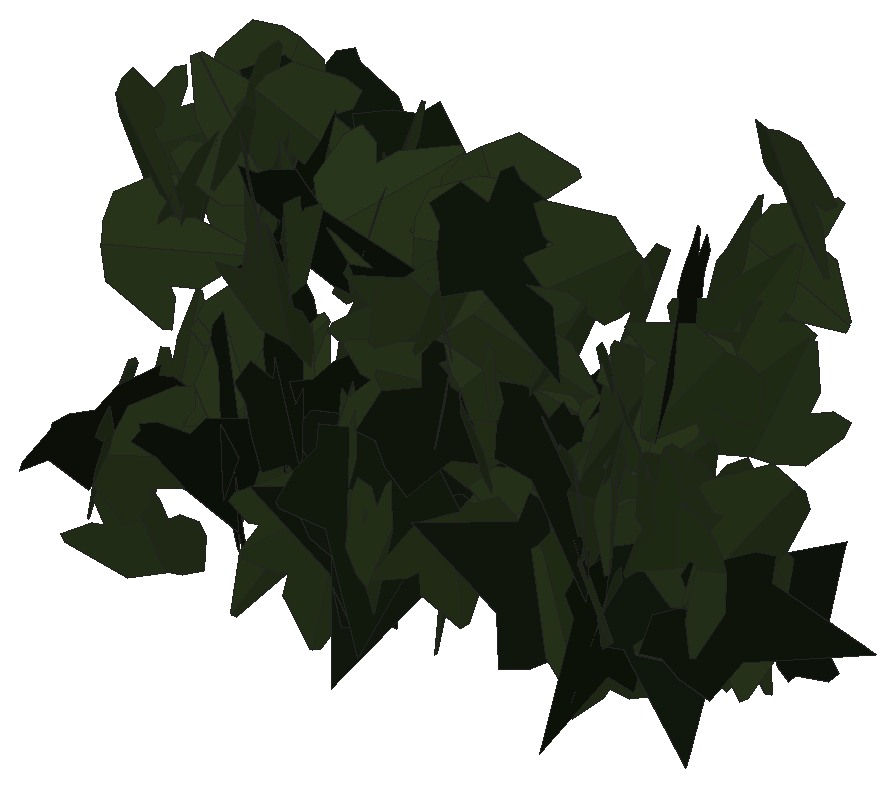
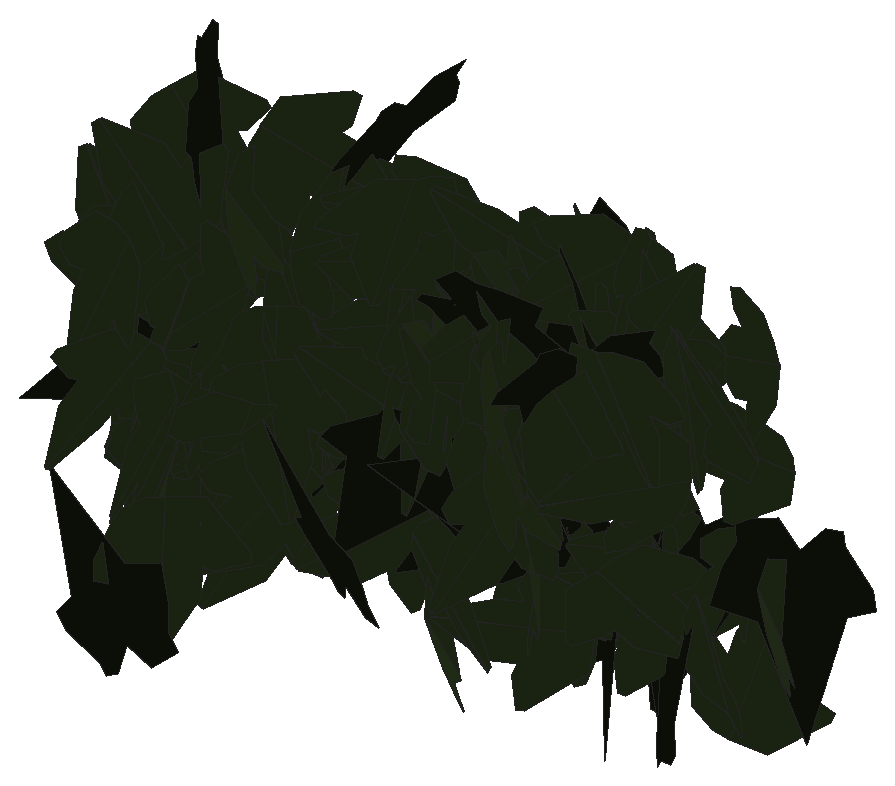
# SketchUp Ruby script. Lengths in inches.
U = 1.inch
M = Sketchup.active_model
def pt(a) = Geom::Point3d.new(a.map { |v| v * U })
def face(e, loops, mat)
  f = e.add_face(loops[0].map { |a| pt(a) })
  loops[1..].each { |l| e.add_face(l.map { |a| pt(a) }).erase! }
  f.material = f.back_material = mat if mat
  f
end
# faces: each face lists its corners as indices into pts; further lists are holes
def faces(e, pts, list, mat = nil) = list.each { |f| face(e, (f[0].is_a?(Array) ? f : [f]).map { |l| l.map { |i| pts[i] } }, mat) }
# xy, xz, yz: faces in a plane at the given z, y or x. An outline is a flat list of corners, or four numbers for a rectangle; further outlines are holes
def ring(l) = l.size == 4 ? [[l[0], l[1]], [l[2], l[1]], [l[2], l[3]], [l[0], l[3]]] : l.each_slice(2).to_a
def flat(e, list, mat, &to3) = list.each { |f| face(e, (f[0].is_a?(Array) ? f : [f]).map { |l| ring(l).map { |u, v| to3.(u, v) } }, mat) }
def xy(e, z, list, mat = nil) = flat(e, list, mat) { |x, y| [x, y, z] }
def xz(e, y, list, mat = nil) = flat(e, list, mat) { |x, z| [x, y, z] }
def yz(e, x, list, mat = nil) = flat(e, list, mat) { |y, z| [x, y, z] }
def lines(e, pts, list) = list.each { |a, b| e.add_line(pt(pts[a]), pt(pts[b])) }
# prism: a flat outline (further loops are holes) pulled along v
def prism(e, loops, v, mat = nil)
  f = face(e, loops, mat); d = Geom::Vector3d.new(v.map { |x| x * U })
  f.pushpull(f.normal.samedirection?(d) ? d.length : -d.length)
end
def box(e, o, s, mat = nil) = prism(e, [[o, [o[0] + s[0], o[1], o[2]], [o[0] + s[0], o[1] + s[1], o[2]], [o[0], o[1] + s[1], o[2]]]], [0, 0, s[2]], mat)
def at(x, y, z, deg = 0) = Geom::Transformation.translation(pt([x, y, z])) * Geom::Transformation.rotation(ORIGIN, Z_AXIS, deg.degrees)
def axes(o, x, y, z) = Geom::Transformation.new([*x, 0, *y, 0, *z, 0, *pt(o).to_a, 1])
def part(name) = M.definitions.add(name)
# library, detail: a bought-in or finely detailed component or shape, given as its bounding box
def library(name, o, s) = part(name).tap { |d| box(d.entities, o, s) }
def detail(e, o, s) = box(e.add_group.entities, o, s)
def put(e, d, t, mat = nil) = e.add_instance(d, t).tap { |i| i.material = mat if mat }
def group(e, t, mat = nil) = e.add_group.tap { |g| g.transformation = t; g.material = mat if mat }.entities
root = M.entities
M.materials.add("efeu1").color = [18, 25, 13]
M.materials.add("efeu2").color = [43, 57, 29]
c1 = part("ivyleaf_9")
p = [[1.54,2.16,1.25],[1.36,2.04,1.19],[-0.21,0.99,0.68],[-0.71,1.11,0.82],[-0.85,0.86,0.67],[-0.8,0.17,0.21],
  [-0.9,-0.01,0.1],[-0.67,-0.16,-0.02],[-0.08,-0.08,-0.05],[-0.03,-0.6,-0.4],[0.65,-0.88,-0.66],[0.83,-0.6,-0.49],
  [1.29,-0.42,-0.43],[1.8125,-0.07,-0.26],[1.21,0.44,0.15]]
faces(c1.entities,p,[[0,1,2,3,4,5,6,7,8,9,10,11,12,13,14]],"efeu1")
c2 = part("ivyleaf_10")
p = [[0,0.5,-0.03],[-0.0625,2.02,-0.43],[-0.19,2.01,-0.46],[-0.54,1.05,-0.29],[-0.52,0.625,-0.18],[-0.83,0.76,-0.28],
  [-1.16,0.64,-0.33],[-1.15,0.33,-0.24],[-0.77,-0.39,0.02],[-0.3,-0.51,0.16],[0.04,-0.48,0.23],[-0.02,2.01,-0.4375],
  [-0.06,2.01,-0.43],[0.04,-0.49,0.23],[0.67,-0.49,0.14],[1.38,0.36,-0.2],[1.375,0.51,-0.24],[0.81,0.65,-0.19],
  [0.62,0.59,-0.15],[0.6,1.09,-0.28],[0.5,1.23,-0.31]]
faces(c2.entities,p,[[0,1,2,3,4,5,6,7,8,9,10],[11,12,0,13,14,15,16,17,18,19,20]],"efeu2")
put(root,c1,axes([20.93,224.31,199.6],[0.02933,0.494,-0.07145],[-0.00437,-0.07131,-0.49487],[-0.49912,0.02966,0.00014]))
put(root,c2,axes([26.3125,224.8,200.39],[-0.04269,-0.38699,-0.31371],[-0.03623,-0.31162,0.38933],[-0.49686,0.05597,-0.00144]))
put(root,c2,axes([24.36,224.5,199.65],[-0.22379,-0.44299,-0.06062],[0.02788,0.05383,-0.49631],[0.44625,-0.22552,0.0006]))
put(root,c2,axes([25.42,224.68,200.18],[-0.3504,0.20605,0.29114],[0.23903,-0.16726,0.40606],[0.26474,0.42375,0.01871]))
put(root,c2,axes([25.79,224.9,201.14],[0.03063,-0.03669,0.49771],[0.24377,-0.43401,-0.047],[0.43547,0.24554,-0.00869]))
put(root,c2,axes([21.23,224.65,198.3125],[-0.46586,-0.11746,-0.13849],[-0.13131,-0.0455,0.4803],[-0.12543,0.48387,0.01154]))
put(root,c2,axes([22.53,224.61,200.82],[-0.48442,0.12063,0.02794],[0.02688,-0.0077,0.49922],[0.12088,0.48517,0.00098]))
put(root,c2,axes([24.4,224.3125,201.29],[0.14748,-0.21102,-0.42862],[-0.16439,0.39877,-0.25289],[0.44858,0.21552,0.04824]))
put(root,c1,axes([23.42,224.79,199.73],[-0.20862,-0.44355,-0.09868],[0.0463,0.08727,-0.49014],[0.45203,-0.21364,0.00466]))
put(root,c2,axes([25.53,224.93,200.15],[0.02152,-0.25545,-0.42928],[0.03012,-0.42823,0.25634],[-0.49863,-0.03689,-0.00304]))
put(root,c2,axes([26.52,224.82,200.34],[-0.13543,-0.42032,-0.23449],[-0.08043,-0.22041,0.44153],[-0.47454,0.15732,-0.00791]))
put(root,c2,axes([23.05,224.64,198.98],[-0.36314,-0.32971,0.09705],[-0.06546,-0.07225,-0.4904],[0.33741,-0.36888,0.00931]))
put(root,c2,axes([25.64,224.79,201.15],[0.00485,-0.06012,0.49635],[0.46659,-0.17781,-0.0261],[0.17965,0.46343,0.05438]))
put(root,c1,axes([23.17,224.91,198.88],[0.14152,-0.47219,-0.08373],[0.02488,-0.07995,0.49294],[-0.47891,-0.14369,0.00086]))
put(root,c2,axes([24.19,224.625,200.46],[-0.44042,-0.15232,0.18119],[0.17046,0.06147,0.46601],[-0.16424,0.47225,-0.00221]))
put(root,c1,axes([25.61,224.9375,199.33],[-0.00761,0.01637,-0.49967],[0.32025,-0.38358,-0.01744],[-0.3839,-0.32031,-0.00465]))
put(root,c2,axes([22.59,224.88,199.08],[-0.10542,-0.36601,0.32392],[-0.04478,-0.32274,-0.37925],[0.4867,-0.10897,0.03527]))
put(root,c2,axes([26.83,224.49,200.18],[0.17159,-0.1198,-0.4541],[-0.37696,0.25321,-0.20924],[0.2801,0.41416,-0.00342]))
put(root,c1,axes([23.45,224.94,199.25],[-0.20647,-0.45045,0.06685],[-0.02706,-0.06113,-0.49551],[0.45458,-0.20823,0.00086]))
put(root,c2,axes([21.29,224.35,199.36],[-0.11899,-0.11951,-0.4707],[0.30395,0.35964,-0.16815],[0.37875,-0.32616,-0.01294]))
put(root,c2,axes([22.99,224.63,199.34],[0.40352,-0.29417,0.02525],[-0.01893,0.01691,0.49936],[-0.29464,-0.40395,0.00251]))
put(root,c2,axes([25.74,224.52,199.41],[-0.28563,0.28325,-0.29696],[-0.21753,0.2023,0.40219],[0.34799,0.35895,0.00767]))
put(root,c1,axes([24.16,224.4,200.88],[0.02505,-0.07182,-0.49418],[0.05742,0.49193,-0.06858],[0.49606,-0.05332,0.03289]))
put(root,c2,axes([24.99,224.79,199.35],[0.33538,-0.07918,0.36229],[0.35486,-0.07332,-0.34452],[0.10768,0.48822,0.00702]))
put(root,c2,axes([25.59,224.83,200.74],[0.35598,-0.21675,0.27621],[0.24827,-0.12274,-0.41629],[0.24826,0.43354,0.02024]))
put(root,c1,axes([21.78,224.47,199.6],[0.33088,0.34787,-0.13967],[-0.1047,-0.09312,-0.47997],[-0.35994,0.34687,0.01122]))
put(root,c1,axes([24.96,224.98,199.14],[0.00282,-0.48119,-0.13581],[0.01758,-0.13563,0.48093],[-0.49968,-0.00749,0.01615]))
put(root,c1,axes([24.55,224.7,202.5],[0.15738,-0.42887,-0.20323],[-0.05426,0.19645,-0.45658],[0.47148,0.16576,0.0153]))
put(root,c1,axes([24.99,224.89,200.65],[0.1566,-0.4703,0.06553],[0.02236,-0.06162,-0.49568],[0.47432,0.15818,0.00173]))
put(root,c2,axes([25.47,224.83,198.82],[0.11892,-0.45782,-0.16203],[0.09079,-0.14292,0.47046],[-0.47709,-0.14132,0.04914]))
put(root,c2,axes([22.71,224.54,201.44],[0.30296,-0.1697,0.35974],[-0.32046,0.16375,0.34712],[-0.23563,-0.44089,-0.00955]))
put(root,c2,axes([20.72,224.89,199.45],[0.25237,-0.39439,0.1754],[0.09208,-0.14932,-0.46822],[0.4217,0.26863,-0.00274]))
put(root,c2,axes([23.65,224.35,199.21],[0.01614,0.1999,-0.45802],[-0.00836,0.4583,0.19973],[0.49967,0.00121,0.01814]))
put(root,c2,axes([26.625,224.85,201.78],[-0.35084,-0.19119,0.30059],[-0.2645,-0.14282,-0.39955],[0.23864,-0.43938,-0.00093]))
put(root,c2,axes([24.6875,224.61,201.55],[-0.30443,-0.19442,-0.34572],[0.28817,0.19105,-0.36119],[0.27254,-0.41917,-0.00427]))
put(root,c2,axes([24.37,224.625,200.66],[-0.29376,0.18589,0.35938],[-0.31475,0.17407,-0.34732],[-0.25424,-0.43029,0.01475]))
put(root,c2,axes([22.29,224.55,201.68],[0.00373,-0.02399,-0.49941],[-0.24123,0.43737,-0.02281],[0.43795,0.24111,-0.00831]))
put(root,c1,axes([22.36,224.9,201.53],[0.25054,-0.13879,0.40984],[0.36925,-0.1783,-0.28611],[0.22557,0.44603,0.01315]))
put(root,c2,axes([23.6,225.1,200.4375],[-0.23494,-0.23039,0.37646],[-0.23923,-0.29192,-0.32795],[0.37091,-0.33422,0.02693]))
put(root,c2,axes([26.93,225.21,200.47],[-0.06618,-0.31554,0.38217],[-0.04541,-0.38008,-0.32168],[0.49352,-0.07728,0.02165]))
put(root,c1,axes([26.03,225.01,199.58],[-0.26778,-0.28128,-0.31492],[0.21339,0.23164,-0.38834],[0.36436,-0.34238,-0.004]))
put(root,c1,axes([22.24,224.93,200.01],[0.29875,-0.36403,-0.16802],[-0.10031,0.135,-0.47086],[0.38818,0.31505,0.00763]))
put(root,c1,axes([26.66,224.65,199.72],[0.06767,0.08338,-0.48833],[0.13967,0.46966,0.09955],[0.4753,-0.14989,0.04027]))
put(root,c2,axes([20.67,225.12,201.8],[-0.15694,0.16078,-0.44668],[0.3258,-0.30571,-0.2245],[-0.34529,-0.36152,-0.00881]))
put(root,c1,axes([21.57,225.26,199.93],[0.09407,-0.0451,-0.489],[0.42853,-0.2356,0.10417],[-0.23982,-0.4387,-0.00567]))
put(root,c2,axes([25.32,225.1875,202.12],[-0.16993,-0.17287,0.43731],[-0.29321,-0.32457,-0.24224],[0.36763,-0.33878,0.00893]))
put(root,c2,axes([20.8,224.95,200.78],[0.07668,-0.07313,-0.48864],[0.49308,-0.02023,0.0804],[-0.03153,-0.49421,0.06901]))
put(root,c2,axes([24.51,224.62,201.125],[0.09999,0.13096,-0.47207],[0.20346,0.42719,0.16161],[0.44565,-0.22441,0.03214]))
put(root,c1,axes([26.16,225.24,202.33],[-0.13376,0.05499,-0.47863],[0.41381,-0.24126,-0.14336],[-0.24671,-0.43448,0.01903]))
put(root,c2,axes([24.21,224.82,201.75],[-0.06656,-0.40781,-0.28153],[0.04846,0.27734,-0.4132],[0.49317,-0.0823,0.00261]))
put(root,c2,axes([23.76,224.91,201.42],[-0.33792,-0.23835,-0.28107],[0.2254,0.16801,-0.41348],[0.29155,-0.40615,-0.0061]))
put(root,c2,axes([26.64,225.39,199.34],[0.0363,0.06567,-0.49434],[-0.32313,-0.37442,-0.07347],[-0.37982,0.32481,0.01526]))
put(root,c2,axes([23.9,224.98,201.89],[-0.02998,-0.02748,-0.49834],[0.4943,0.06741,-0.03345],[0.06903,-0.49467,0.02313]))
put(root,c2,axes([24.02,225.07,200.9375],[-0.164,-0.04741,-0.46995],[0.47221,-0.02819,-0.16194],[-0.01114,-0.49695,0.05402]))
put(root,c2,axes([24.86,225.48,201.48],[0.03531,-0.13844,0.47915],[0.2077,-0.43264,-0.14031],[0.45345,0.20895,0.02696]))
put(root,c2,axes([21.98,225.17,200.38],[0.47383,-0.05811,-0.14869],[-0.14751,0.01871,-0.47738],[0.06104,0.49626,0.00058]))
put(root,c2,axes([22.99,224.98,201.82],[0.30132,0.00592,-0.39897],[0.38725,0.11614,0.29419],[0.09616,-0.48629,0.0654]))
put(root,c1,axes([21.9375,225.24,200.71],[-0.21749,-0.02532,-0.44951],[0.44516,0.06253,-0.21891],[0.0673,-0.49543,-0.00465]))
put(root,c2,axes([25.8,225.37,199.8],[-0.16367,-0.37558,0.28661],[-0.09581,-0.27064,-0.40936],[0.46264,-0.18892,0.01663]))
put(root,c2,axes([24.45,225.24,199.38],[0.41401,-0.0476,0.27628],[0.27321,-0.04193,-0.41665],[0.06283,0.49596,-0.0087]))
put(root,c1,axes([23.08,225.08,199.24],[-0.29452,0.10518,0.39012],[0.36057,-0.14945,0.3125],[0.18235,0.4654,0.01218]))
put(root,c2,axes([21.7,225.2,199.16],[-0.00883,0.01404,-0.49972],[0.49121,-0.09264,-0.01128],[-0.09291,-0.49114,-0.01215]))
put(root,c2,axes([26.01,225.25,201.44],[0.42027,0.23542,-0.13399],[-0.12261,-0.05521,-0.48158],[-0.24154,0.43764,0.01132]))
put(root,c2,axes([24.35,225.01,199.96],[-0.17604,-0.29383,0.36424],[0.178,0.31787,0.34245],[-0.43281,0.25024,-0.00732]))
put(root,c2,axes([22.78,225.05,199.21],[0.08107,-0.03634,-0.49204],[-0.40145,0.28501,-0.08719],[0.28681,0.4092,0.01703]))
put(root,c2,axes([25.45,225.2,200.35],[-0.36013,-0.34649,-0.01594],[0.01161,0.01092,-0.49975],[0.34666,-0.36031,0.00018]))
put(root,c2,axes([25.52,225.03,198.8125],[-0.18617,-0.29451,-0.35862],[0.17493,0.31335,-0.34815],[0.42981,-0.2551,-0.01363]))
put(root,c2,axes([21.29,225.27,201.64],[0.09345,-0.48409,-0.08323],[-0.0203,0.08085,-0.493],[0.49077,0.09552,-0.00455]))
put(root,c1,axes([22.875,225.13,199.85],[0.01317,-0.13391,-0.48155],[0.23515,0.42674,-0.11224],[0.44106,-0.22352,0.07422]))
put(root,c2,axes([23.99,225.11,200.87],[-0.07812,-0.38304,-0.31173],[0.06265,0.30537,-0.39093],[0.48987,-0.10014,0.00029]))
put(root,c1,axes([22.17,225.09,199.3],[0.14723,0.0017,-0.47783],[-0.46258,0.12581,-0.14208],[0.11975,0.48391,0.03862]))
put(root,c2,axes([23,225.59,200.51],[-0.08661,-0.39415,0.2952],[-0.01435,-0.29759,-0.40154],[0.49223,-0.07803,0.04024]))
put(root,c2,axes([21.6875,225.36,201.6],[0.3291,0.31938,0.19922],[-0.14236,-0.13936,0.4586],[0.34846,-0.35857,-0.00079]))
put(root,c2,axes([25.35,225.05,199.49],[-0.09308,-0.06818,-0.48651],[0.34657,0.34182,-0.11421],[0.34817,-0.35848,-0.01637]))
put(root,c1,axes([22.73,225.16,199.75],[0.18047,0.01494,0.46606],[0.46253,0.05763,-0.18095],[-0.05913,0.49644,0.00698]))
put(root,c2,axes([22.01,225.29,202.28],[-0.30895,-0.04588,-0.39045],[0.39046,0.02198,-0.31154],[0.04575,-0.49741,0.02224]))
put(root,c2,axes([25.625,225.4,199.62],[0.09981,-0.06472,-0.48564],[0.4734,-0.11494,0.11261],[-0.12621,-0.48229,0.03833]))
put(root,c1,axes([22.4,225.07,201.73],[-0.26657,0.13879,-0.3996],[-0.36814,0.15652,0.29995],[0.20835,0.45413,0.01874]))
put(root,c2,axes([21.78,225.01,199.64],[0.16541,0.16316,-0.44274],[0.18539,0.40895,0.21997],[0.4339,-0.23693,0.07479]))
put(root,c1,axes([21.57,225.25,198.45],[0.09781,-0.23107,0.43248],[-0.09755,0.42302,0.24808],[-0.48054,-0.1329,0.03767]))
put(root,c2,axes([25.4,225.65,201.76],[0.17218,-0.35775,0.30392],[0.14859,-0.26554,-0.39675],[0.44528,0.22694,0.01487]))
put(root,c2,axes([20.59,225.54,201.34],[0.19967,-0.18155,-0.42092],[0.35913,-0.22337,0.26671],[-0.28488,-0.40883,0.0412]))
put(root,c2,axes([21.77,225.16,202.26],[0.00033,-0.34073,-0.36593],[-0.00405,0.36591,-0.34072],[0.49998,0.00319,-0.00252]))
put(root,c2,axes([26.43,225.39,199.6],[0.12969,-0.02539,-0.48222],[-0.46798,0.11651,-0.13199],[0.11907,0.48557,0.00645]))
put(root,c2,axes([24.08,225.38,199.3],[-0.30916,-0.01579,-0.39265],[0.39234,0.01583,-0.30955],[0.02221,-0.4995,0.0026]))
put(root,c1,axes([23.82,225.44,200.09],[-0.14035,-0.23731,-0.41712],[0.21118,0.35971,-0.2757],[0.43094,-0.25356,-0.00074]))
put(root,c2,axes([22.53,225.27,198.79],[0.05758,0.0325,-0.49561],[0.43919,0.22965,0.06609],[0.23193,-0.44295,-0.0021]))
put(root,c2,axes([22.94,225.37,201.49],[0.18122,-0.38497,0.2626],[-0.12941,0.22909,0.42517],[-0.44767,-0.22207,-0.01661]))
put(root,c2,axes([23.94,225.46,202.23],[0.20335,0.44546,0.10108],[0.0434,0.0913,-0.48967],[-0.45472,0.20792,-0.00153]))
put(root,c2,axes([23.33,225.81,198.78],[0.26893,-0.2584,0.33303],[0.23036,-0.24073,-0.3728],[0.353,0.35395,-0.01043]))
put(root,c2,axes([23.11,225.52,201.11],[0.2842,-0.35479,-0.20821],[-0.13994,0.15459,-0.45444],[0.38684,0.31658,-0.01143]))
put(root,c2,axes([26.59,225.57,200.81],[-0.31372,-0.36511,0.13517],[0.08766,0.10289,0.48138],[-0.37933,0.32574,-0.00055]))
put(root,c2,axes([25.26,225.57,200.08],[-0.45078,-0.14495,0.1606],[-0.15139,-0.05381,-0.47348],[0.15454,-0.4755,0.00462]))
put(root,c2,axes([23.27,225.9,200.96],[-0.05558,-0.29803,0.3976],[-0.02362,-0.39805,-0.30166],[0.49634,-0.05232,0.03017]))
put(root,c2,axes([20.78,225.53,198.99],[0.46147,-0.18728,0.04446],[-0.03358,0.0354,0.49761],[-0.18953,-0.46225,0.0201]))
put(root,c2,axes([23.01,225.29,201.46],[-0.08619,-0.14571,-0.47047],[0.28672,0.3735,-0.1682],[0.40046,-0.29878,0.01917]))
put(root,c2,axes([26.21,225.64,198.84],[-0.22976,0.43018,0.11024],[0.04877,-0.09893,0.48768],[0.4414,0.23485,0.0035]))
put(root,c2,axes([25.125,225.48,199.24],[-0.33624,-0.15644,-0.33537],[0.30851,0.13175,-0.37077],[0.20437,-0.45626,0.00793]))
put(root,c2,axes([23.69,225.51,200.65],[-0.42327,0.25353,0.08102],[-0.07093,0.03926,-0.49338],[-0.25654,-0.42916,0.00273]))
put(root,c1,axes([23.12,225.8,201.76],[-0.47717,-0.04147,0.14348],[-0.1419,-0.02404,-0.47884],[0.04662,-0.4977,0.01117]))
put(root,c2,axes([26.17,226.01,201.14],[-0.08971,-0.16255,-0.46425],[-0.21091,-0.41361,0.18558],[-0.44437,0.22913,0.00564]))
put(root,c2,axes([23.22,225.57,201.05],[-0.34593,0.2547,-0.25585],[-0.20797,0.14906,0.42957],[0.2951,0.40362,0.00282]))
put(root,c2,axes([21.97,225.32,201.42],[0.04823,-0.10497,0.48647],[-0.1919,0.44703,0.11548],[-0.45918,-0.19784,0.00283]))
put(root,c2,axes([21.5,225.84,199.82],[0.33482,0.20912,-0.30686],[-0.25881,-0.16488,-0.39475],[-0.2663,0.42318,-0.00217]))
put(root,c2,axes([22.7,225.43,199.37],[0.04429,0.00383,0.49802],[-0.4022,0.29515,0.0335],[-0.29373,-0.40357,0.02922]))
put(root,c2,axes([25.39,225.64,199.82],[0.3432,0.33166,0.14905],[0.10298,0.1079,-0.47723],[-0.34872,0.35828,0.00575]))
put(root,c2,axes([26.12,225.71,199.34],[-0.46471,0.15417,-0.10137],[0.09113,-0.04709,-0.48936],[-0.16044,-0.4733,0.01567]))
put(root,c2,axes([22.45,226.03,200.67],[0.10271,-0.42479,0.2429],[0.04789,-0.23828,-0.43696],[0.48699,0.11303,-0.00827]))
put(root,c2,axes([26.1,225.73,201.42],[-0.24331,-0.37417,0.22539],[0.11594,0.19342,0.44626],[-0.42114,0.26942,-0.00736]))
put(root,c2,axes([22.625,225.91,201.28],[0.13668,-0.48088,-0.00835],[-0.00278,0.00789,-0.49993],[0.48095,0.13671,-0.00052]))
put(root,c2,axes([23.38,225.71,200.85],[0.21092,-0.37688,0.25194],[-0.12511,0.21869,0.43188],[-0.43573,-0.24522,-0.00205]))
put(root,c2,axes([25.7,225.5,200.78],[0.03525,-0.05384,0.49584],[-0.16686,0.46716,0.06259],[-0.47002,-0.16989,0.01497]))
put(root,c2,axes([22.11,225.93,201.07],[-0.20132,-0.01807,0.45732],[-0.45325,-0.06149,-0.20195],[0.06354,-0.49588,0.00838]))
put(root,c2,axes([23.32,225.875,199.44],[0.24658,-0.18333,-0.39445],[-0.31712,0.23458,-0.30726],[0.29772,0.4017,-0.00059]))
put(root,c2,axes([22.63,225.79,200.125],[-0.17793,-0.30593,-0.3532],[0.17122,0.30896,-0.35387],[0.43477,-0.24687,-0.00518]))
put(root,c1,axes([21.625,226.17,201.92],[-0.03846,-0.43951,-0.23527],[0.03306,0.2332,-0.44105],[0.49742,-0.04948,0.01112]))
put(root,c2,axes([21.25,226.24,201.96],[0.48778,-0.05407,-0.09562],[-0.0948,0.01263,-0.49077],[0.05549,0.49691,0.00207]))
put(root,c2,axes([21.55,226.39,201.53],[-0.18472,-0.40464,0.22834],[-0.09677,-0.20684,-0.44481],[0.45444,-0.20853,-0.0019]))
put(root,c2,axes([25.72,226.24,199.01],[-0.30709,-0.393,-0.03531],[0.02141,0.02808,-0.49875],[0.394,-0.30784,-0.00042]))
put(root,c2,axes([21.07,225.91,200.91],[-0.00878,-0.04937,0.49748],[0.10638,0.48598,0.05011],[-0.48847,0.10673,0.00197]))
put(root,c1,axes([23.94,226.25,199.21],[-0.21314,0.3106,0.32878],[0.18526,-0.27162,0.3767],[0.41261,0.2824,0.0007]))
put(root,c1,axes([25.71,226.75,198.29],[-0.16301,0.06176,0.46863],[0.3327,-0.33713,0.16016],[0.33576,0.36404,0.06882]))
put(root,c2,axes([25.46,226.47,201.17],[-0.1484,0.25784,0.40187],[-0.21262,0.34112,-0.29737],[-0.42752,-0.25915,0.0084]))
put(root,c2,axes([25.3125,227.4,202.0625],[-0.42519,0.22217,-0.14091],[0.12171,-0.07131,-0.47969],[-0.23324,-0.44222,0.00656]))
put(root,c2,axes([25.21,227.34,201.16],[0.06164,0.36563,0.33543],[0.04926,0.33183,-0.37076],[-0.49373,0.07876,0.00488]))
put(root,c2,axes([24.875,227.37,200.77],[-0.07714,0.13716,0.47459],[-0.23305,0.41343,-0.15737],[-0.43559,-0.24549,0.00014]))
